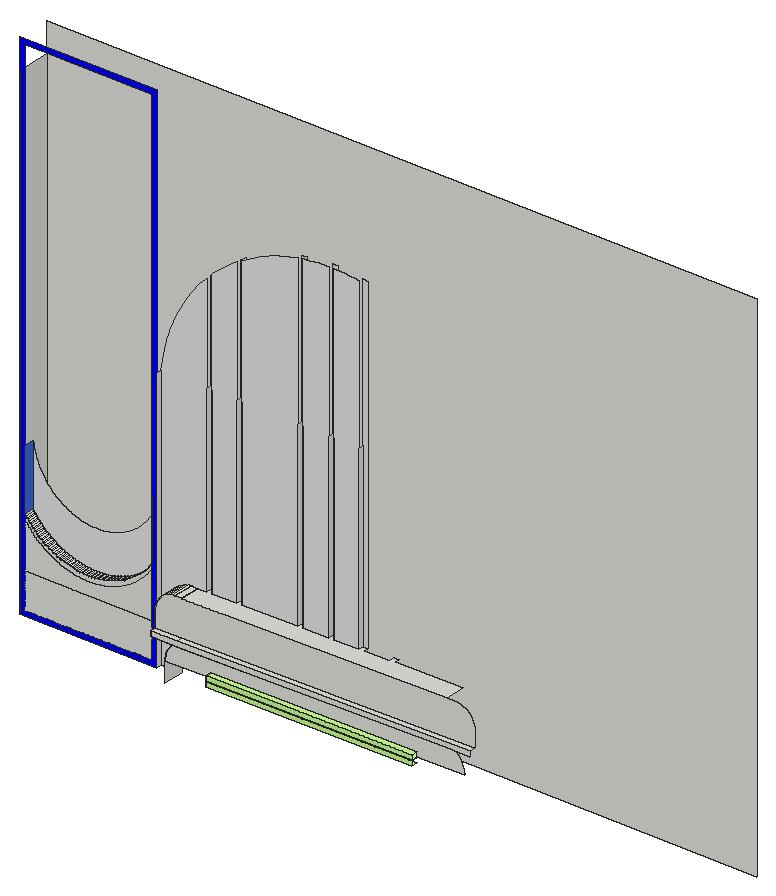
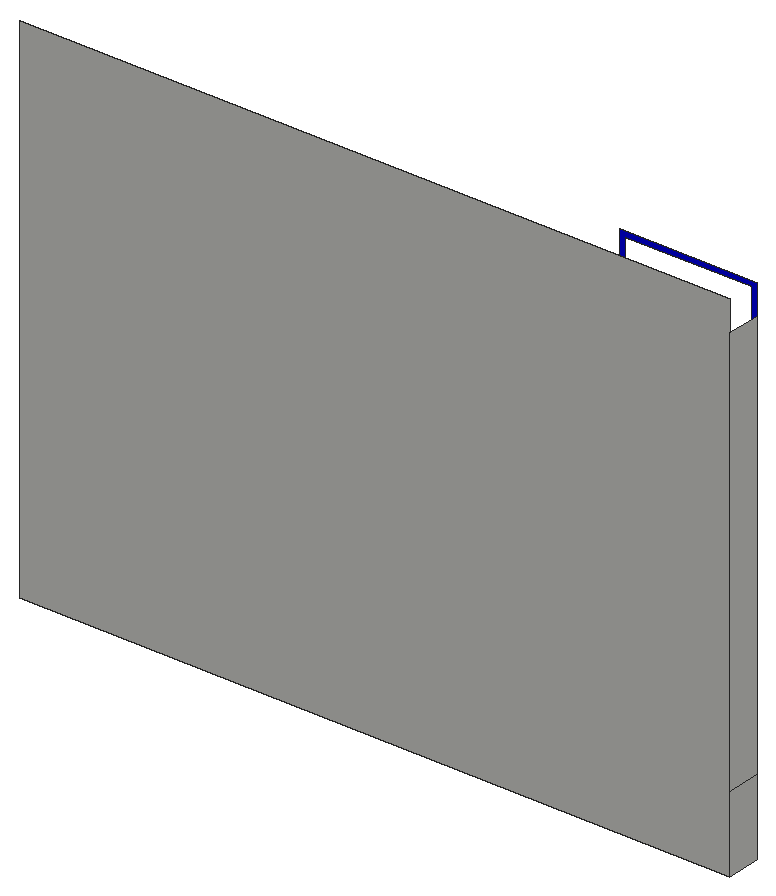
# SketchUp Ruby script. Lengths in inches.
U = 1.inch
M = Sketchup.active_model
def pt(a) = Geom::Point3d.new(a.map { |v| v * U })
def face(e, loops, mat)
  f = e.add_face(loops[0].map { |a| pt(a) })
  loops[1..].each { |l| e.add_face(l.map { |a| pt(a) }).erase! }
  f.material = f.back_material = mat if mat
  f
end
# faces: each face lists its corners as indices into pts; further lists are holes
def faces(e, pts, list, mat = nil) = list.each { |f| face(e, (f[0].is_a?(Array) ? f : [f]).map { |l| l.map { |i| pts[i] } }, mat) }
# xy, xz, yz: faces in a plane at the given z, y or x. An outline is a flat list of corners, or four numbers for a rectangle; further outlines are holes
def ring(l) = l.size == 4 ? [[l[0], l[1]], [l[2], l[1]], [l[2], l[3]], [l[0], l[3]]] : l.each_slice(2).to_a
def flat(e, list, mat, &to3) = list.each { |f| face(e, (f[0].is_a?(Array) ? f : [f]).map { |l| ring(l).map { |u, v| to3.(u, v) } }, mat) }
def xy(e, z, list, mat = nil) = flat(e, list, mat) { |x, y| [x, y, z] }
def xz(e, y, list, mat = nil) = flat(e, list, mat) { |x, z| [x, y, z] }
def yz(e, x, list, mat = nil) = flat(e, list, mat) { |y, z| [x, y, z] }
def lines(e, pts, list) = list.each { |a, b| e.add_line(pt(pts[a]), pt(pts[b])) }
# prism: a flat outline (further loops are holes) pulled along v
def prism(e, loops, v, mat = nil)
  f = face(e, loops, mat); d = Geom::Vector3d.new(v.map { |x| x * U })
  f.pushpull(f.normal.samedirection?(d) ? d.length : -d.length)
end
def box(e, o, s, mat = nil) = prism(e, [[o, [o[0] + s[0], o[1], o[2]], [o[0] + s[0], o[1] + s[1], o[2]], [o[0], o[1] + s[1], o[2]]]], [0, 0, s[2]], mat)
def at(x, y, z, deg = 0) = Geom::Transformation.translation(pt([x, y, z])) * Geom::Transformation.rotation(ORIGIN, Z_AXIS, deg.degrees)
def axes(o, x, y, z) = Geom::Transformation.new([*x, 0, *y, 0, *z, 0, *pt(o).to_a, 1])
def part(name) = M.definitions.add(name)
# library, detail: a bought-in or finely detailed component or shape, given as its bounding box
def library(name, o, s) = part(name).tap { |d| box(d.entities, o, s) }
def detail(e, o, s) = box(e.add_group.entities, o, s)
def put(e, d, t, mat = nil) = e.add_instance(d, t).tap { |i| i.material = mat if mat }
def group(e, t, mat = nil) = e.add_group.tap { |g| g.transformation = t; g.material = mat if mat }.entities
root = M.entities
M.materials.add("[0102_RoyalBlue]").color = [65, 105, 225]
M.materials.add("[0103_Blue]").color = [0, 0, 255]
M.materials.add("[Aluminum]").color = [229, 229, 229]
M.materials.add("[Color F02]").color = [204, 255, 153]
xy(root,8.108,[[29,0.125,31.874,5.25],[31.874,0.125,34.207,6.25]])
xy(root,9.108,[[29,0.125,34.207,1.25]])
xy(root,11.438,[[13.352,4.25,13.648,6.25]])
xy(root,16.11,[[33,1.25,34.207,5.25]])
xz(root,0,[[40.112,3.073,80.688,3.396,80.688,4.296,40.104,3.973],[40.104,4.173,80.6875,4.496,80.688,5.396,40.123,5.073,40.096,5.072]],"[Color F02]")
xz(root,0.125,[[29,8.108,34.207,8.108,86.574,8.889,88.696,8.921,92,8.97,92,9.97,34.207,9.108,29,9.108]])
xz(root,1.25,[[31,4,40.104,4.073,40.104,4.173,40.096,5.072,40.123,5.073,80.688,5.396,80.6875,4.496,80.688,4.396,90,4.47,89.972,4.971,89.89,5.465,89.889,5.469,89.754,5.948,89.566,6.412,89.328,6.853,89.043,7.266,88.715,7.645,88.347,7.985,87.944,8.283,87.51,8.535,87.052,8.738,86.574,8.889,34.207,8.108,33.76,7.969,33.331,7.783,32.926,7.55,32.549,7.274,32.204,6.958,31.897,6.605,31.63,6.222,31.407,5.811,31.23,5.378,31.124,5.001,31.103,4.928,31.026,4.467],[29,9.108,34.207,9.108,92,9.97,92,12.97,91.966,13.489,91.863,14,91.695,14.492,91.462,14.957,91.171,15.389,91,15.581,90.825,15.777,90.431,16.117,90,16.4,89.996,16.402,89.527,16.628,89.032,16.789,88.52,16.884,88.001,16.91,86.574,16.889,34.207,16.108,34.207,16.11,33,16.11,33,16.108,32.478,16.073,31.965,15.971,31.469,15.803,31,15.572,30.565,15.281,30.172,14.936,29.827,14.543,29.536,14.108,29.304,13.638,29.136,13.143,29.034,12.63,29,12.108]])
xz(root,4.25,[[1,1,26,8],[1,8,26,8,26,17,25.829,16.757,25.654,16.518,25.473,16.283,25.289,16.051,25.1,15.822,24.906,15.598,24.708,15.377,24.506,15.16,24.299,14.947,24.089,14.738,23.874,14.533,23.655,14.333,23.433,14.136,23.207,13.945,22.977,13.757,22.743,13.574,22.506,13.396,22.265,13.223,22.021,13.054,21.774,12.89,21.524,12.731,21.271,12.576,21.014,12.427,20.755,12.283,20.493,12.144,20.229,12.01,19.961,11.881,19.692,11.757,19.42,11.639,19.145,11.526,18.869,11.418,18.591,11.316,18.31,11.219,18.028,11.128,17.744,11.043,17.458,10.962,17.171,10.888,16.883,10.819,16.593,10.756,16.302,10.698,16.01,10.646,15.717,10.6,15.423,10.56,15.128,10.525,14.833,10.496,14.537,10.473,14.241,10.456,13.945,10.444,13.648,10.438,13.352,10.438,13.055,10.444,12.759,10.456,12.463,10.473,12.167,10.496,11.872,10.525,11.577,10.56,11.283,10.6,10.99,10.646,10.698,10.698,10.407,10.756,10.117,10.819,9.829,10.888,9.542,10.962,9.256,11.043,8.972,11.128,8.69,11.219,8.409,11.316,8.131,11.418,7.855,11.526,7.58,11.639,7.308,11.757,7.039,11.881,6.771,12.01,6.507,12.144,6.245,12.283,5.986,12.427,5.729,12.576,5.476,12.731,5.226,12.89,4.979,13.054,4.735,13.223,4.494,13.396,4.257,13.574,4.023,13.757,3.793,13.945,3.567,14.136,3.345,14.333,3.126,14.533,2.911,14.738,2.701,14.947,2.494,15.16,2.292,15.377,2.094,15.598,1.9,15.822,1.711,16.051,1.527,16.283,1.346,16.518,1.171,16.757,1,17],[13.352,10.438,13.648,10.438,13.945,10.444,14.241,10.456,14.537,10.473,14.833,10.496,15.128,10.525,15.423,10.56,15.717,10.6,16.01,10.646,16.302,10.698,16.593,10.756,16.883,10.819,17.171,10.888,17.458,10.962,17.744,11.043,18.028,11.128,18.31,11.219,18.591,11.316,18.869,11.418,19.145,11.526,19.42,11.639,19.692,11.757,19.961,11.881,20.229,12.01,20.493,12.144,20.755,12.283,21.014,12.427,21.271,12.576,21.524,12.731,21.774,12.89,22.021,13.054,22.265,13.223,22.506,13.396,22.743,13.574,22.977,13.757,23.207,13.945,23.433,14.136,23.655,14.333,23.874,14.533,24.089,14.738,24.299,14.947,24.506,15.16,24.708,15.377,24.906,15.598,25.1,15.822,25.289,16.051,25.473,16.283,25.654,16.518,25.829,16.757,26,17,26,18,25.829,17.757,25.654,17.518,25.473,17.283,25.289,17.051,25.1,16.822,24.906,16.598,24.708,16.377,24.506,16.16,24.299,15.947,24.089,15.738,23.874,15.533,23.655,15.333,23.433,15.136,23.207,14.945,22.977,14.757,22.743,14.574,22.506,14.396,22.265,14.223,22.021,14.054,21.774,13.89,21.524,13.731,21.271,13.576,21.014,13.427,20.755,13.283,20.493,13.144,20.229,13.01,19.961,12.881,19.692,12.757,19.42,12.639,19.145,12.526,18.869,12.418,18.591,12.316,18.31,12.219,18.028,12.128,17.744,12.043,17.458,11.962,17.171,11.888,16.883,11.819,16.593,11.756,16.302,11.698,16.01,11.646,15.717,11.6,15.423,11.56,15.128,11.525,14.833,11.496,14.537,11.473,14.241,11.456,13.945,11.444,13.648,11.438,13.352,11.438,13.055,11.444,12.759,11.456,12.463,11.473,12.167,11.496,11.872,11.525,11.577,11.56,11.283,11.6,10.99,11.646,10.698,11.698,10.407,11.756,10.117,11.819,9.829,11.888,9.542,11.962,9.256,12.043,8.972,12.128,8.69,12.219,8.409,12.316,8.131,12.418,7.855,12.526,7.58,12.639,7.308,12.757,7.039,12.881,6.771,13.01,6.507,13.144,6.245,13.283,5.986,13.427,5.729,13.576,5.476,13.731,5.226,13.89,4.979,14.054,4.735,14.223,4.494,14.396,4.257,14.574,4.023,14.757,3.793,14.945,3.567,15.136,3.345,15.333,3.126,15.533,2.911,15.738,2.701,15.947,2.494,16.16,2.292,16.377,2.094,16.598,1.9,16.822,1.711,17.051,1.527,17.283,1.346,17.518,1.171,17.757,1,18,1,17,1.171,16.757,1.346,16.518,1.527,16.283,1.711,16.051,1.9,15.822,2.094,15.598,2.292,15.377,2.494,15.16,2.701,14.947,2.911,14.738,3.126,14.533,3.345,14.333,3.567,14.136,3.793,13.945,4.023,13.757,4.257,13.574,4.494,13.396,4.735,13.223,4.979,13.054,5.226,12.89,5.476,12.731,5.729,12.576,5.986,12.427,6.245,12.283,6.507,12.144,6.771,12.01,7.039,11.881,7.308,11.757,7.58,11.639,7.855,11.526,8.131,11.418,8.409,11.316,8.69,11.219,8.972,11.128,9.256,11.043,9.542,10.962,9.829,10.888,10.117,10.819,10.407,10.756,10.698,10.698,10.99,10.646,11.283,10.6,11.577,10.56,11.872,10.525,12.167,10.496,12.463,10.473,12.759,10.456,13.055,10.444]])
xz(root,4.25,[[[0,0,27,102],[1,1,26,101]]],"[0103_Blue]")
xz(root,5.25,[[27,0,31,0,31,4,31.026,4.467,31.103,4.928,31.124,5.001,31.23,5.378,31.407,5.811,31.63,6.222,31.897,6.605,31.874,8.108,29,8.108,29,12.108,29.034,12.63,29.136,13.143,29.304,13.638,29.536,14.108,29.827,14.543,30.172,14.936,30.565,15.281,31,15.572,31.469,15.803,31.965,15.971,32.478,16.073,33,16.108,33,16.11,34.207,16.11,34.207,16.108,36,16.134,36,71.44,35.38,70.767,34.728,70.016,34.098,69.246,33.492,68.458,32.909,67.653,32.35,66.83,31.815,65.992,31.305,65.138,30.821,64.269,30.363,63.386,29.931,62.491,29.525,61.582,29.147,60.663,28.795,59.732,28.472,58.792,28.176,57.842,28.162,57.792,27.909,56.885,27.669,55.919,27.459,54.947,27.277,53.969,27.124,52.987,27,52],[37,16.149,42,16.224,42,76.466,41.332,76.019,40.523,75.441,39.731,74.84,38.956,74.216,38.201,73.569,37.465,72.9,37,72.451],[43,16.239,54,16.403,54,81.366,53.102,81.178,52.135,80.945,51.175,80.684,50.223,80.395,49.281,80.078,48.348,79.733,47.426,79.361,46.515,78.962,45.616,78.536,44.73,78.083,43.859,77.605,43.001,77.101,43,77.101],[55,16.418,60,16.493,60,81.996,59.009,81.967,58.016,81.908,57.025,81.82,56.038,81.703,55.054,81.557,55,81.547],[61,16.507,66,16.582,66,81.547,65.946,81.557,64.962,81.703,63.975,81.82,62.984,81.908,61.991,81.967,61,81.996]],"[Aluminum]")
xz(root,6.25,[[40.104,3.973,42,3.988,42,4.088,40.104,4.073],[42,3.988,54,4.083,54,4.183,42,4.088],[40.104,4.073,42,4.088,42,4.1875,40.104,4.173],[54,4.083,60,4.131,60,4.231,54,4.183],[42,4.088,54,4.183,54,4.283,42,4.1875],
  [60,4.131,66,4.179,66,4.279,60,4.231],[54,4.183,60,4.231,60,4.331,54,4.283],[60,4.231,66,4.279,66,4.379,60,4.331],[31.897,6.605,32.204,6.958,32.549,7.274,32.926,7.55,33.331,7.783,33.76,7.969,34.207,8.108,31.874,8.108],[36,16.134,37,16.149,37,72.451,36.749,72.21,36.054,71.499,36,71.44],
  [42,16.224,43,16.239,43,77.101,42.159,76.572,42,76.466],[54,16.403,55,16.418,55,81.547,54.075,81.382,54,81.366],[60,16.493,61,16.507,61,81.996,60,81.996],[66,16.582,67,16.597,67,81.366,66.925,81.382,66,81.547]])
xz(root,6.25,[[13.352,11.438,13.648,11.438,13.945,11.444,14.241,11.456,14.537,11.473,14.833,11.496,15.128,11.525,15.423,11.56,15.717,11.6,16.01,11.646,16.302,11.698,16.593,11.756,16.883,11.819,17.171,11.888,17.458,11.962,17.744,12.043,18.028,12.128,18.31,12.219,18.591,12.316,18.869,12.418,19.145,12.526,19.42,12.639,19.692,12.757,19.961,12.881,20.229,13.01,20.493,13.144,20.755,13.283,21.014,13.427,21.271,13.576,21.524,13.731,21.774,13.89,22.021,14.054,22.265,14.223,22.506,14.396,22.743,14.574,22.977,14.757,23.207,14.945,23.433,15.136,23.655,15.333,23.874,15.533,24.089,15.738,24.299,15.947,24.506,16.16,24.708,16.377,24.906,16.598,25.1,16.822,25.289,17.051,25.473,17.283,25.654,17.518,25.829,17.757,26,18,26,30,25.95,29.635,25.889,29.271,25.818,28.91,25.736,28.55,25.643,28.193,25.54,27.839,25.427,27.489,25.304,27.141,25.17,26.798,25.027,26.458,24.873,26.123,24.71,25.793,24.537,25.467,24.355,25.146,24.164,24.831,23.963,24.522,23.753,24.219,23.535,23.922,23.308,23.632,23.073,23.348,22.829,23.071,22.577,22.802,22.318,22.54,22.051,22.286,21.777,22.039,21.496,21.801,21.207,21.571,20.913,21.35,20.611,21.138,20.304,20.934,19.991,20.739,19.673,20.554,19.349,20.378,19.02,20.212,18.686,20.055,18.348,19.908,18.006,19.771,17.66,19.644,17.31,19.528,16.957,19.421,16.601,19.325,16.243,19.24,15.882,19.165,15.519,19.1,15.154,19.047,14.788,19.004,14.421,18.971,14.053,18.95,13.684,18.939,13.316,18.939,12.947,18.95,12.579,18.971,12.212,19.004,11.846,19.047,11.481,19.1,11.118,19.165,10.757,19.24,10.399,19.325,10.043,19.421,9.69,19.528,9.34,19.644,8.994,19.771,8.652,19.908,8.314,20.055,7.98,20.212,7.651,20.378,7.327,20.554,7.009,20.739,6.696,20.934,6.389,21.138,6.087,21.35,5.793,21.571,5.504,21.801,5.223,22.039,4.949,22.286,4.682,22.54,4.423,22.802,4.171,23.071,3.927,23.348,3.692,23.632,3.465,23.922,3.247,24.219,3.037,24.522,2.836,24.831,2.645,25.146,2.463,25.467,2.29,25.793,2.127,26.123,1.973,26.458,1.83,26.798,1.696,27.141,1.573,27.489,1.46,27.839,1.357,28.193,1.264,28.55,1.182,28.91,1.111,29.271,1.05,29.635,1,30,1,18,1.171,17.757,1.346,17.518,1.527,17.283,1.711,17.051,1.9,16.822,2.094,16.598,2.292,16.377,2.494,16.16,2.701,15.947,2.911,15.738,3.126,15.533,3.345,15.333,3.567,15.136,3.793,14.945,4.023,14.757,4.257,14.574,4.494,14.396,4.735,14.223,4.979,14.054,5.226,13.89,5.476,13.731,5.729,13.576,5.986,13.427,6.245,13.283,6.507,13.144,6.771,13.01,7.039,12.881,7.308,12.757,7.58,12.639,7.855,12.526,8.131,12.418,8.409,12.316,8.69,12.219,8.972,12.128,9.256,12.043,9.542,11.962,9.829,11.888,10.117,11.819,10.407,11.756,10.698,11.698,10.99,11.646,11.283,11.6,11.577,11.56,11.872,11.525,12.167,11.496,12.463,11.473,12.759,11.456,13.055,11.444]],"[Aluminum]")
xz(root,10.75,[[0,0,140,102]])
yz(root,0,[[4.25,0,10.75,15],[4.25,15,10.75,96]])
yz(root,1,[[4.25,18,6.25,30]],"[0102_RoyalBlue]")
yz(root,26,[[4.25,18,6.25,30]],"[0102_RoyalBlue]")
yz(root,27,[[4.25,0,5.25,52]])
yz(root,29,[[0.125,8.108,5.25,9.108],[1.25,9.108,5.25,12.108]])
yz(root,31,[[1.25,0,5.25,4]])
yz(root,33,[[1.25,16.108,5.25,16.11]])
yz(root,34.207,[[1.25,16.108,5.25,16.11]])
yz(root,36,[[5.25,16.134,6.25,52]])
yz(root,37,[[5.25,16.149,6.25,52]])
yz(root,40.104,[[1.25,3.973,6.25,4.073],[1.25,4.073,6.25,4.173]])
yz(root,42,[[5.25,16.224,6.25,52]])
yz(root,43,[[5.25,16.239,6.25,52]])
yz(root,54,[[5.25,16.403,6.25,52]])
yz(root,55,[[5.25,16.418,6.25,52]])
yz(root,60,[[5.25,16.493,6.25,52]])
yz(root,61,[[5.25,16.507,6.25,52]])
yz(root,66,[[5.25,16.582,6.25,52]])
p = [[40.112,0,3.073],[40.104,0,3.973],[40.104,1.25,3.973],[40.112,1.25,3.073],[80.688,0,3.396],[80.688,1.25,3.396],
  [42,6.25,3.988],[40.104,6.25,3.973],[80.688,0,4.296],[80.688,1.25,4.296],[80.688,6.25,4.296],[72,6.25,4.227],
  [66,6.25,4.179],[60,6.25,4.131],[54,6.25,4.083],[31.026,5.25,4.467],[31,5.25,4],[31,1.25,4],
  [31.026,1.25,4.467],[40.104,0,4.173],[40.096,0,5.072],[40.096,1.25,5.072],[40.104,1.25,4.173],[40.104,6.25,4.173],
  [42,6.25,4.1875],[54,6.25,4.283],[60,6.25,4.331],[66,6.25,4.379],[72,6.25,4.427],[80.6875,6.25,4.496],
  [80.6875,1.25,4.496],[80.6875,0,4.496],[31.103,5.25,4.928],[31.103,1.25,4.928],[31.124,5.25,5.001],[31.124,1.25,5.001],
  [31.23,5.25,5.378],[31.23,1.25,5.378],[40.123,0,5.073],[40.123,1.25,5.073],[80.688,0,5.396],[80.688,1.25,5.396],
  [31.407,5.25,5.811],[31.407,1.25,5.811],[31.63,5.25,6.222],[31.63,1.25,6.222],[31.897,5.25,6.605],[31.897,1.25,6.605],
  [32.204,6.25,6.958],[31.897,6.25,6.605],[32.204,1.25,6.958],[31.874,6.25,8.108],[31.874,5.25,8.108],[32.549,6.25,7.274],
  [32.549,1.25,7.274],[32.926,6.25,7.55],[32.926,1.25,7.55],[33.331,6.25,7.783],[33.331,1.25,7.783],[33.76,6.25,7.969],
  [33.76,1.25,7.969],[34.207,6.25,8.108],[34.207,1.25,8.108],[86.574,1.25,8.889],[86.574,0.125,8.889],[34.207,0.125,8.108],
  [92,1.25,9.97],[34.207,1.25,9.108],[34.207,0.125,9.108],[92,0.125,9.97],[13.055,6.25,11.444],[12.759,6.25,11.456],
  [12.759,4.25,11.456],[13.055,4.25,11.444],[13.352,6.25,11.438],[13.352,4.25,11.438],[13.945,6.25,11.444],[13.648,6.25,11.438],
  [13.648,4.25,11.438],[13.945,4.25,11.444],[14.241,6.25,11.456],[14.241,4.25,11.456],[11.872,6.25,11.525],[11.577,6.25,11.56],
  [11.577,4.25,11.56],[11.872,4.25,11.525],[12.167,6.25,11.496],[12.167,4.25,11.496],[12.463,6.25,11.473],[12.463,4.25,11.473],
  [14.537,6.25,11.473],[14.537,4.25,11.473],[14.833,6.25,11.496],[14.833,4.25,11.496],[15.128,6.25,11.525],[15.128,4.25,11.525],
  [15.423,6.25,11.56],[15.423,4.25,11.56],[10.99,6.25,11.646],[10.698,6.25,11.698],[10.698,4.25,11.698],[10.99,4.25,11.646],
  [11.283,6.25,11.6],[11.283,4.25,11.6],[15.717,6.25,11.6],[15.717,4.25,11.6],[16.01,6.25,11.646],[16.01,4.25,11.646],
  [16.302,6.25,11.698],[16.302,4.25,11.698],[10.407,6.25,11.756],[10.407,4.25,11.756],[16.593,6.25,11.756],[16.593,4.25,11.756],
  [10.117,6.25,11.819],[9.829,6.25,11.888],[9.829,4.25,11.888],[10.117,4.25,11.819],[16.883,6.25,11.819],[16.883,4.25,11.819],
  [17.171,6.25,11.888],[17.171,4.25,11.888],[9.542,6.25,11.962],[9.542,4.25,11.962],[17.458,6.25,11.962],[17.458,4.25,11.962],
  [9.256,6.25,12.043],[8.972,6.25,12.128],[8.972,4.25,12.128],[9.256,4.25,12.043],[17.744,6.25,12.043],[17.744,4.25,12.043],
  [18.028,6.25,12.128],[18.028,4.25,12.128],[29.034,5.25,12.63],[29,5.25,12.108],[29,1.25,12.108],[29.034,1.25,12.63],
  [8.69,6.25,12.219],[8.69,4.25,12.219],[18.31,6.25,12.219],[18.31,4.25,12.219],[8.409,6.25,12.316],[8.409,4.25,12.316],
  [18.591,6.25,12.316],[18.591,4.25,12.316],[8.131,6.25,12.418],[8.131,4.25,12.418],[18.869,6.25,12.418],[18.869,4.25,12.418],
  [7.855,6.25,12.526],[7.855,4.25,12.526],[19.145,6.25,12.526],[19.145,4.25,12.526],[7.58,6.25,12.639],[7.58,4.25,12.639],
  [19.42,6.25,12.639],[19.42,4.25,12.639],[29.136,5.25,13.143],[29.136,1.25,13.143],[7.308,6.25,12.757],[7.308,4.25,12.757],
  [19.692,6.25,12.757],[19.692,4.25,12.757],[7.039,6.25,12.881],[7.039,4.25,12.881],[19.961,6.25,12.881],[19.961,4.25,12.881],
  [6.771,6.25,13.01],[6.771,4.25,13.01],[20.229,6.25,13.01],[20.229,4.25,13.01],[6.507,6.25,13.144],[6.507,4.25,13.144],
  [20.493,6.25,13.144],[20.493,4.25,13.144],[29.304,5.25,13.638],[29.304,1.25,13.638],[6.245,6.25,13.283],[6.245,4.25,13.283],
  [20.755,6.25,13.283],[20.755,4.25,13.283],[5.986,6.25,13.427],[5.986,4.25,13.427],[21.014,6.25,13.427],[21.014,4.25,13.427],
  [5.729,6.25,13.576],[5.729,4.25,13.576],[21.271,6.25,13.576],[21.271,4.25,13.576],[29.536,5.25,14.108],[29.536,1.25,14.108],
  [5.476,6.25,13.731],[5.476,4.25,13.731],[21.524,6.25,13.731],[21.524,4.25,13.731],[5.226,6.25,13.89],[5.226,4.25,13.89],
  [21.774,6.25,13.89],[21.774,4.25,13.89],[4.979,6.25,14.054],[4.979,4.25,14.054],[22.021,6.25,14.054],[22.021,4.25,14.054],
  [29.827,5.25,14.543],[29.827,1.25,14.543],[4.735,6.25,14.223],[4.735,4.25,14.223],[22.265,6.25,14.223],[22.265,4.25,14.223],
  [4.494,6.25,14.396],[4.494,4.25,14.396],[22.506,6.25,14.396],[22.506,4.25,14.396],[4.257,6.25,14.574],[4.257,4.25,14.574],
  [22.743,6.25,14.574],[22.743,4.25,14.574],[30.172,5.25,14.936],[30.172,1.25,14.936],[4.023,6.25,14.757],[4.023,4.25,14.757],
  [22.977,6.25,14.757],[22.977,4.25,14.757],[3.793,6.25,14.945],[3.793,4.25,14.945],[23.207,6.25,14.945],[23.207,4.25,14.945],
  [30.565,5.25,15.281],[30.565,1.25,15.281],[3.567,6.25,15.136],[3.567,4.25,15.136],[23.433,6.25,15.136],[23.433,4.25,15.136],
  [3.345,6.25,15.333],[3.345,4.25,15.333],[23.655,6.25,15.333],[23.655,4.25,15.333],[31,5.25,15.572],[31,1.25,15.572],
  [3.126,6.25,15.533],[3.126,4.25,15.533],[23.874,6.25,15.533],[23.874,4.25,15.533],[2.911,6.25,15.738],[2.911,4.25,15.738],
  [24.089,6.25,15.738],[24.089,4.25,15.738],[31.469,5.25,15.803],[31.469,1.25,15.803],[2.701,6.25,15.947],[2.701,4.25,15.947],
  [24.299,6.25,15.947],[24.299,4.25,15.947],[31.965,5.25,15.971],[31.965,1.25,15.971],[2.494,6.25,16.16],[2.494,4.25,16.16],
  [24.506,6.25,16.16],[24.506,4.25,16.16],[32.478,5.25,16.073],[32.478,1.25,16.073],[33,5.25,16.108],[33,1.25,16.108],
  [36,6.25,16.134],[36,5.25,16.134],[34.207,5.25,16.108],[34.207,1.25,16.108],[86.574,1.25,16.889],[86.574,5.25,16.889],
  [73,5.25,16.687],[73,6.25,16.687],[72,6.25,16.672],[72,5.25,16.672],[67,5.25,16.597],[67,6.25,16.597],
  [66,6.25,16.582],[66,5.25,16.582],[61,5.25,16.507],[61,6.25,16.507],[60,6.25,16.493],[60,5.25,16.493],
  [55,5.25,16.418],[55,6.25,16.418],[54,6.25,16.403],[54,5.25,16.403],[43,5.25,16.239],[43,6.25,16.239],
  [42,6.25,16.224],[42,5.25,16.224],[37,5.25,16.149],[37,6.25,16.149],[2.292,6.25,16.377],[2.292,4.25,16.377],
  [24.708,6.25,16.377],[24.708,4.25,16.377],[2.094,6.25,16.598],[2.094,4.25,16.598],[24.906,6.25,16.598],[24.906,4.25,16.598],
  [1.9,6.25,16.822],[1.9,4.25,16.822],[25.1,6.25,16.822],[25.1,4.25,16.822],[1.711,6.25,17.051],[1.711,4.25,17.051],
  [25.289,6.25,17.051],[25.289,4.25,17.051],[1.527,6.25,17.283],[1.527,4.25,17.283],[25.473,6.25,17.283],[25.473,4.25,17.283],
  [1.346,6.25,17.518],[1.346,4.25,17.518],[25.654,6.25,17.518],[25.654,4.25,17.518],[1.171,6.25,17.757],[1.171,4.25,17.757],
  [25.829,6.25,17.757],[25.829,4.25,17.757],[1,6.25,18],[1,4.25,18],[26,6.25,18],[26,4.25,18],
  [42,6.25,3.088],[42,6.25,5.088],[54,6.25,5.088],[54,6.25,3.988],[54,6.25,3.183],[54,6.25,4.04],
  [54,6.25,3.088],[54,6.25,5.183],[60,6.25,5.088],[60,6.25,4.088],[60,6.25,4.083],[60,6.25,5.183],
  [60,6.25,3.183],[60,6.25,3.088],[60,6.25,4.04],[60,6.25,3.988],[60,6.25,3.231],[60,6.25,5.231],
  [66,6.25,5.183],[66,6.25,5.088],[66,6.25,3.183],[66,6.25,3.088],[66,6.25,4.083],[66,6.25,4.04],
  [66,6.25,3.988],[66,6.25,3.279],[66,6.25,4.088],[66,6.25,5.231],[66,6.25,4.131],[66,6.25,3.231],
  [66,6.25,5.279],[37,6.25,16.134],[61,6.25,16.493],[55,6.25,16.403],[43,6.25,16.224]]
faces(root,p,[[0,1,2,3],[4,0,3,5],[6,7,2,1,8,9,10,11,12,13,14],[19,20,21,22],[23,24,25,26,27,28,29,30,31,19,22],[38,40,41,39]],"[Color F02]")
faces(root,p,[[15,16,17,18],[32,15,18,33],[34,32,33,35],[36,34,35,37],[20,38,39,21],[42,36,37,43],[44,42,43,45],[46,44,45,47],
  [48,49,46,47,50],[49,51,52,46],[53,48,50,54],[55,53,54,56],[57,55,56,58],[59,57,58,60],[61,59,60,62],[62,63,64,65],
  [66,67,68,69],[70,71,72,73],[74,70,73,75],[76,77,78,79],[80,76,79,81],[82,83,84,85],[86,82,85,87],[88,86,87,89],
  [71,88,89,72],[90,80,81,91],[92,90,91,93],[94,92,93,95],[96,94,95,97],[98,99,100,101],[102,98,101,103],[83,102,103,84],
  [104,96,97,105],[106,104,105,107],[108,106,107,109],[99,110,111,100],[112,108,109,113],[114,115,116,117],[110,114,117,111],[118,112,113,119],
  [120,118,119,121],[115,122,123,116],[124,120,121,125],[126,127,128,129],[122,126,129,123],[130,124,125,131],[132,130,131,133],[134,135,136,137],
  [127,138,139,128],[140,132,133,141],[138,142,143,139],[144,140,141,145],[142,146,147,143],[148,144,145,149],[146,150,151,147],[152,148,149,153],
  [150,154,155,151],[156,152,153,157],[158,134,137,159],[154,160,161,155],[162,156,157,163],[160,164,165,161],[166,162,163,167],[164,168,169,165],
  [170,166,167,171],[168,172,173,169],[174,170,171,175],[176,158,159,177],[172,178,179,173],[180,174,175,181],[178,182,183,179],[184,180,181,185],
  [182,186,187,183],[188,184,185,189],[190,176,177,191],[186,192,193,187],[194,188,189,195],[192,196,197,193],[198,194,195,199],[196,200,201,197],
  [202,198,199,203],[204,190,191,205],[200,206,207,201],[208,202,203,209],[206,210,211,207],[212,208,209,213],[210,214,215,211],[216,212,213,217],
  [218,204,205,219],[214,220,221,215],[222,216,217,223],[220,224,225,221],[226,222,223,227],[228,218,219,229],[224,230,231,225],[232,226,227,233],
  [230,234,235,231],[236,232,233,237],[238,228,229,239],[234,240,241,235],[242,236,237,243],[240,244,245,241],[246,242,243,247],[248,238,239,249],
  [244,250,251,245],[252,246,247,253],[254,248,249,255],[250,256,257,251],[258,252,253,259],[260,254,255,261],[262,260,261,263],[264,265,266,267,268,269,270,271,272,273,274,275,276,277,278,279,280,281,282,283,284,285,286,287,288,289,290,291],
  [256,292,293,257],[294,258,259,295],[292,296,297,293],[298,294,295,299],[296,300,301,297],[302,298,299,303],[300,304,305,301],[306,302,303,307],
  [304,308,309,305],[310,306,307,311],[308,312,313,309],[314,310,311,315],[312,316,317,313],[318,314,315,319],[316,320,321,317],[322,318,319,323]])
lines(root,p,[[6,324],[325,24],[326,25],[327,328],[329,327],[14,329],[328,330],[331,326],[332,26],[333,334],[335,332],[336,337],
  [334,338],[339,340],[338,339],[13,333],[340,336],[341,335],[342,343],[344,345],[346,347],[348,349],[343,27],[350,346],
  [347,348],[351,342],[352,350],[353,344],[12,352],[354,351],[349,353],[291,355],[279,356],[283,357],[287,358]])
